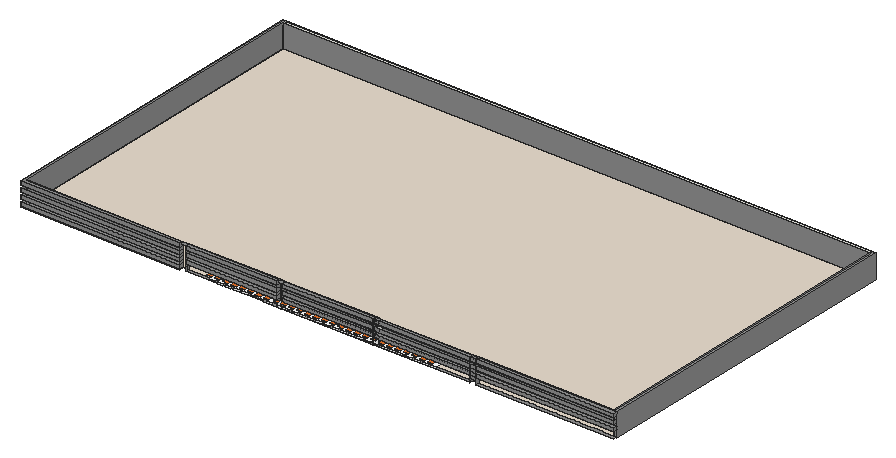
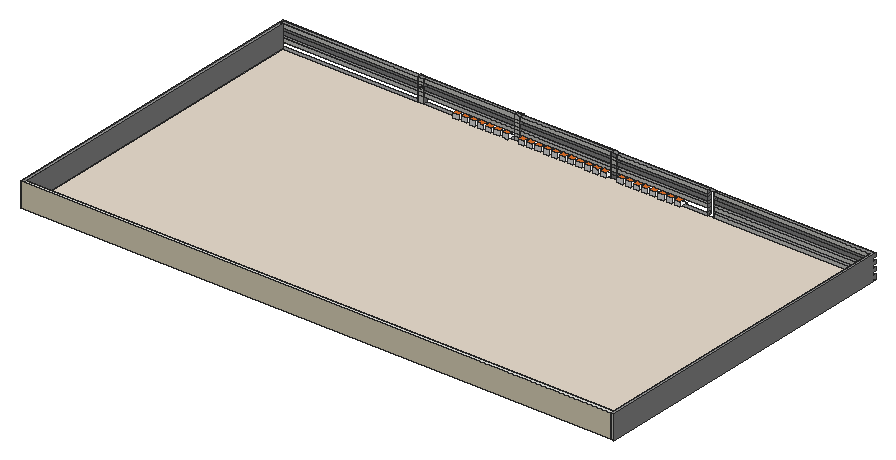
# SketchUp Ruby script. Lengths in inches.
U = 1.inch
M = Sketchup.active_model
def pt(a) = Geom::Point3d.new(a.map { |v| v * U })
def face(e, loops, mat)
  f = e.add_face(loops[0].map { |a| pt(a) })
  loops[1..].each { |l| e.add_face(l.map { |a| pt(a) }).erase! }
  f.material = f.back_material = mat if mat
  f
end
# faces: each face lists its corners as indices into pts; further lists are holes
def faces(e, pts, list, mat = nil) = list.each { |f| face(e, (f[0].is_a?(Array) ? f : [f]).map { |l| l.map { |i| pts[i] } }, mat) }
# xy, xz, yz: faces in a plane at the given z, y or x. An outline is a flat list of corners, or four numbers for a rectangle; further outlines are holes
def ring(l) = l.size == 4 ? [[l[0], l[1]], [l[2], l[1]], [l[2], l[3]], [l[0], l[3]]] : l.each_slice(2).to_a
def flat(e, list, mat, &to3) = list.each { |f| face(e, (f[0].is_a?(Array) ? f : [f]).map { |l| ring(l).map { |u, v| to3.(u, v) } }, mat) }
def xy(e, z, list, mat = nil) = flat(e, list, mat) { |x, y| [x, y, z] }
def xz(e, y, list, mat = nil) = flat(e, list, mat) { |x, z| [x, y, z] }
def yz(e, x, list, mat = nil) = flat(e, list, mat) { |y, z| [x, y, z] }
def lines(e, pts, list) = list.each { |a, b| e.add_line(pt(pts[a]), pt(pts[b])) }
# prism: a flat outline (further loops are holes) pulled along v
def prism(e, loops, v, mat = nil)
  f = face(e, loops, mat); d = Geom::Vector3d.new(v.map { |x| x * U })
  f.pushpull(f.normal.samedirection?(d) ? d.length : -d.length)
end
def box(e, o, s, mat = nil) = prism(e, [[o, [o[0] + s[0], o[1], o[2]], [o[0] + s[0], o[1] + s[1], o[2]], [o[0], o[1] + s[1], o[2]]]], [0, 0, s[2]], mat)
def at(x, y, z, deg = 0) = Geom::Transformation.translation(pt([x, y, z])) * Geom::Transformation.rotation(ORIGIN, Z_AXIS, deg.degrees)
def axes(o, x, y, z) = Geom::Transformation.new([*x, 0, *y, 0, *z, 0, *pt(o).to_a, 1])
def part(name) = M.definitions.add(name)
# library, detail: a bought-in or finely detailed component or shape, given as its bounding box
def library(name, o, s) = part(name).tap { |d| box(d.entities, o, s) }
def detail(e, o, s) = box(e.add_group.entities, o, s)
def put(e, d, t, mat = nil) = e.add_instance(d, t).tap { |i| i.material = mat if mat }
def group(e, t, mat = nil) = e.add_group.tap { |g| g.transformation = t; g.material = mat if mat }.entities
root = M.entities
M.materials.add("Generic").color = [146, 146, 146]
M.materials.add("Generic\#3").color = [226, 112, 41]
M.materials.add("Generic\#5").color = [249, 239, 211]
M.materials.add("Generic\#7").color = [232, 220, 205]
M.materials.add("[Color M00]").color = [255, 255, 255]
xy(root,1896.75,[[1505.875,322,1513,1033.625],[217.0625,1025.625,1505.875,1033.625]])
xy(root,1896.75,[[209.5,313.625,560.3,322],[209.5,322,217.0625,1033.625]],"Generic")
xy(root,1898.5625,[[773.9375,313.625,780.55,322]],"Generic")
xy(root,1899.375,[[572.47,313.625,737.9375,313.625,737.9375,314.3125,744.55,314.3125,744.55,313.625,772.57,313.625,772.57,322,572.47,322],[784.74,313.625,984.84,322],[997.01,313.625,1197.11,322],[1209.29,313.625,1513,322]],"Generic")
xy(root,1899.375,[[217.0625,322,1505.875,1025.625]],"Generic\#7")
xy(root,1902.875,[[624.9375,313.625,636.55,333.5625],[642.9375,313.625,654.55,333.5625],[660.9375,313.625,672.55,333.5625],[678.9375,313.625,690.55,333.5625],[696.9375,313.625,708.55,333.5625],
  [714.9375,313.625,726.55,333.5625],[732.9375,313.625,744.55,333.5625],[750.9375,313.625,762.55,333.5625],[786.9375,313.625,798.55,333.5625],[804.9375,313.625,816.55,333.5625],
  [822.9375,313.625,834.55,333.5625],[840.9375,313.625,852.55,333.5625],[858.9375,313.625,870.55,333.5625],[876.9375,313.625,888.55,333.5625],[894.9375,313.625,906.55,333.5625],
  [912.9375,313.625,924.55,333.5625],[930.9375,313.625,942.55,333.5625],[948.9375,313.625,960.55,333.5625],[966.9375,313.625,978.55,333.5625],[1002.9375,313.625,1014.55,333.5625],
  [1020.9375,313.625,1032.55,333.5625],[1038.9375,313.625,1050.55,333.5625],[1056.9375,313.625,1068.55,333.5625],[1074.9375,313.625,1086.55,333.5625],[1092.9375,313.625,1104.55,333.5625],
  [1110.9375,313.625,1122.55,333.5625]],"[Color M00]")
xy(root,1907.375,[[209.5,313.625,560.3,322]],"Generic")
xy(root,1913.3125,[[209.5,313.625,560.3,322],[572.47,313.625,624.9375,322],[624.9375,313.625,636.55,322],[636.55,313.625,642.9375,322],[642.9375,313.625,654.55,322],
  [654.55,313.625,660.9375,322],[660.9375,313.625,672.55,322],[672.55,313.625,678.9375,322],[678.9375,313.625,690.55,322],[690.55,313.625,696.9375,322],
  [696.9375,313.625,708.55,322],[708.55,313.625,714.9375,322],[714.9375,313.625,726.55,322],[726.55,313.625,732.9375,322],[732.9375,313.625,744.55,322],
  [744.55,313.625,750.9375,322],[750.9375,313.625,762.55,322],[762.55,313.625,772.57,322],[784.74,313.625,786.9375,322],[786.9375,313.625,798.55,322],
  [798.55,313.625,804.9375,322],[804.9375,313.625,816.55,322],[816.55,313.625,822.9375,322],[822.9375,313.625,834.55,322],[834.55,313.625,840.9375,322],
  [840.9375,313.625,852.55,322],[852.55,313.625,858.9375,322],[858.9375,313.625,870.55,322],[870.55,313.625,876.9375,322],[876.9375,313.625,888.55,322],
  [888.55,313.625,894.9375,322],[894.9375,313.625,906.55,322],[906.55,313.625,912.9375,322],[912.9375,313.625,924.55,322],[924.55,313.625,930.9375,322],
  [930.9375,313.625,942.55,322],[942.55,313.625,948.9375,322],[948.9375,313.625,960.55,322],[960.55,313.625,966.9375,322],[966.9375,313.625,978.55,322],
  [978.55,313.625,1002.9375,322],[1002.9375,313.625,1014.55,322],[1014.55,313.625,1020.9375,322],[1020.9375,313.625,1032.55,322],[1032.55,313.625,1038.9375,322],
  [1038.9375,313.625,1050.55,322],[1050.55,313.625,1056.9375,322],[1056.9375,313.625,1068.55,322],[1068.55,313.625,1074.9375,322],[1074.9375,313.625,1086.55,322],
  [1086.55,313.625,1092.9375,322],[1092.9375,313.625,1104.55,322],[1104.55,313.625,1110.9375,322],[1110.9375,313.625,1122.55,322],[1122.55,313.625,1513,322]],"Generic")
xy(root,1913.3125,[[732.9375,303.9375,744.55,313.625],[624.9375,305.625,636.55,313.625],[642.9375,305.625,654.55,313.625],[660.9375,305.625,672.55,313.625],[678.9375,305.625,690.55,313.625],
  [696.9375,305.625,708.55,313.625],[714.9375,305.625,726.55,313.625],[750.9375,305.625,762.55,313.625],[772.57,305.625,780.55,313.625],[786.9375,305.625,798.55,313.625],
  [804.9375,305.625,816.55,313.625],[822.9375,305.625,834.55,313.625],[840.9375,305.625,852.55,313.625],[858.9375,305.625,870.55,313.625],[876.9375,305.625,888.55,313.625],
  [894.9375,305.625,906.55,313.625],[912.9375,305.625,924.55,313.625],[930.9375,305.625,942.55,313.625],[948.9375,305.625,960.55,313.625],[966.9375,305.625,978.55,313.625],
  [984.9375,305.625,996.55,312.1875],[1002.9375,305.625,1014.55,313.625],[1020.9375,305.625,1032.55,313.625],[1038.9375,305.625,1050.55,313.625],[1056.9375,305.625,1068.55,313.625],
  [1074.9375,305.625,1086.55,313.625],[1092.9375,305.625,1104.55,313.625],[1110.9375,305.625,1122.55,313.625],[624.9375,322,636.55,333.5625],[642.9375,322,654.55,333.5625],
  [660.9375,322,672.55,333.5625],[678.9375,322,690.55,333.5625],[696.9375,322,708.55,333.5625],[714.9375,322,726.55,333.5625],[732.9375,322,744.55,333.5625],
  [750.9375,322,762.55,333.5625],[786.9375,322,798.55,333.5625],[804.9375,322,816.55,333.5625],[822.9375,322,834.55,333.5625],[840.9375,322,852.55,333.5625],
  [858.9375,322,870.55,333.5625],[876.9375,322,888.55,333.5625],[894.9375,322,906.55,333.5625],[912.9375,322,924.55,333.5625],[930.9375,322,942.55,333.5625],
  [948.9375,322,960.55,333.5625],[966.9375,322,978.55,333.5625],[1002.9375,322,1014.55,333.5625],[1020.9375,322,1032.55,333.5625],[1038.9375,322,1050.55,333.5625],
  [1056.9375,322,1068.55,333.5625],[1074.9375,322,1086.55,333.5625],[1092.9375,322,1104.55,333.5625],[1110.9375,322,1122.55,333.5625]],"Generic\#3")
xy(root,1921.3125,[[209.5,313.625,560.3,322],[572.47,313.625,772.57,322],[784.74,313.625,1513,322]],"Generic")
xy(root,1927.25,[[209.5,313.625,560.3,322],[572.47,313.625,772.57,322],[784.74,313.625,1513,322]],"Generic")
xy(root,1941.1875,[[209.5,313.625,560.3,322],[572.47,313.625,772.57,322],[784.74,313.625,1513,322]],"Generic")
xy(root,1949.1875,[[217.0625,1025.625,1505.875,1033.625]])
xy(root,1949.1875,[[984.84,312.1875,997.01,313.625],[1197.11,312.6875,1209.29,313.625],[209.5,313.625,560.3,313.625,560.3,322,217.0625,322,217.0625,1033.625,209.5,1033.625],[560.3,313.625,572.47,322],[572.47,313.625,772.57,322],
  [772.57,313.625,784.74,322],[784.74,313.625,984.84,322],[984.84,313.625,997.01,322],[997.01,313.625,1197.11,322],[1197.11,313.625,1209.29,322],
  [1209.29,313.625,1513,322],[1505.875,322,1513,1033.625]],"Generic")
xz(root,312.1875,[[984.9375,1902.875,996.55,1913.3125]],"[Color M00]")
xz(root,313.625,[[209.5,1899.375,560.3,1907.375],[984.84,1899.375,997.01,1907.375],[984.84,1907.375,997.01,1913.3125],[1197.11,1907.375,1209.29,1913.3125],[209.5,1913.3125,560.3,1921.3125],
  [572.47,1913.3125,772.57,1921.3125],[784.74,1913.3125,984.84,1921.3125],[984.84,1913.3125,997.01,1921.3125],[997.01,1913.3125,1197.11,1921.3125],[1197.11,1913.3125,1209.29,1921.3125],
  [1209.29,1913.3125,1513,1921.3125],[1197.11,1921.3125,1209.29,1927.25],[209.5,1927.25,560.3,1935.25],[572.47,1927.25,772.57,1935.25],[784.74,1927.25,984.84,1935.25],
  [984.84,1927.25,997.01,1935.25],[997.01,1927.25,1197.11,1935.25],[1197.11,1927.25,1209.29,1935.25],[1209.29,1927.25,1513,1935.25],[209.5,1941.1875,560.3,1949.1875],
  [572.47,1941.1875,772.57,1949.1875],[784.74,1941.1875,984.84,1949.1875],[984.84,1941.1875,997.01,1949.1875],[997.01,1941.1875,1197.11,1949.1875],[1197.11,1941.1875,1209.29,1949.1875],
  [1209.29,1941.1875,1513,1949.1875]],"Generic")
xz(root,313.625,[[772.57,1898.5625,780.55,1902.875],[624.9375,1899.375,636.55,1902.875],[642.9375,1899.375,654.55,1902.875],[660.9375,1899.375,672.55,1902.875],[678.9375,1899.375,690.55,1902.875],
  [696.9375,1899.375,708.55,1902.875],[714.9375,1899.375,726.55,1902.875],[750.9375,1899.375,762.55,1902.875],[786.9375,1899.375,798.55,1902.875],[804.9375,1899.375,816.55,1902.875],
  [822.9375,1899.375,834.55,1902.875],[840.9375,1899.375,852.55,1902.875],[858.9375,1899.375,870.55,1902.875],[876.9375,1899.375,888.55,1902.875],[894.9375,1899.375,906.55,1902.875],
  [912.9375,1899.375,924.55,1902.875],[930.9375,1899.375,942.55,1902.875],[948.9375,1899.375,960.55,1902.875],[966.9375,1899.375,978.55,1902.875],[1002.9375,1899.375,1014.55,1902.875],
  [1020.9375,1899.375,1032.55,1902.875],[1038.9375,1899.375,1050.55,1902.875],[1056.9375,1899.375,1068.55,1902.875],[1074.9375,1899.375,1086.55,1902.875],[1092.9375,1899.375,1104.55,1902.875],
  [1110.9375,1899.375,1122.55,1902.875],[772.57,1902.875,780.55,1913.3125]],"[Color M00]")
xz(root,322,[[217.0625,1899.375,560.3,1907.375],[984.84,1899.375,997.01,1907.375],[1197.11,1899.375,1209.29,1913.3125],[984.84,1907.375,997.01,1913.3125],[217.0625,1913.3125,560.3,1921.3125],
  [572.47,1913.3125,772.57,1921.3125],[772.57,1913.3125,784.74,1921.3125],[784.74,1913.3125,984.84,1921.3125],[984.84,1913.3125,997.01,1921.3125],[997.01,1913.3125,1197.11,1921.3125],
  [1197.11,1913.3125,1209.29,1921.3125],[1197.11,1913.3125,1209.29,1935.25],[1209.29,1913.3125,1505.875,1921.3125],[1505.875,1913.3125,1513,1921.3125],[984.84,1921.3125,997.01,1927.25],
  [984.84,1921.3125,997.01,1935.25],[1197.11,1921.3125,1209.29,1927.25],[772.57,1927.25,784.74,1935.25],[984.84,1927.25,997.01,1935.25],[1197.11,1927.25,1209.29,1935.25],
  [772.57,1935.25,784.74,1941.1875],[984.84,1935.25,997.01,1941.1875],[1197.11,1935.25,1209.29,1941.1875],[217.0625,1941.1875,560.3,1949.1875],[572.47,1941.1875,772.57,1949.1875],
  [784.74,1941.1875,984.84,1949.1875],[984.84,1941.1875,997.01,1949.1875],[997.01,1941.1875,1197.11,1949.1875],[1197.11,1941.1875,1209.29,1949.1875],[1209.29,1941.1875,1505.875,1949.1875],
  [1505.875,1941.1875,1513,1949.1875]])
xz(root,322,[[209.5,1896.75,217.0625,1899.375],[1505.875,1896.75,1513,1899.375],[772.57,1899.375,784.74,1907.375],[1505.875,1899.375,1513,1913.3125],[209.5,1907.375,217.0625,1913.3125],
  [772.57,1907.375,784.74,1913.3125],[209.5,1921.3125,217.0625,1927.25],[772.57,1921.3125,784.74,1927.25],[1505.875,1921.3125,1513,1927.25],[217.0625,1927.25,560.3,1935.25],
  [572.47,1927.25,772.57,1935.25],[784.74,1927.25,984.84,1935.25],[997.01,1927.25,1197.11,1935.25],[1209.29,1927.25,1505.875,1935.25],[1505.875,1927.25,1513,1941.1875],
  [209.5,1935.25,217.0625,1941.1875],[772.57,1941.1875,784.74,1949.1875]],"Generic")
xz(root,333.5625,[[624.9375,1902.875,636.55,1913.3125],[642.9375,1902.875,654.55,1913.3125],[660.9375,1902.875,672.55,1913.3125],[678.9375,1902.875,690.55,1913.3125],[696.9375,1902.875,708.55,1913.3125],
  [714.9375,1902.875,726.55,1913.3125],[732.9375,1902.875,744.55,1913.3125],[750.9375,1902.875,762.55,1913.3125],[786.9375,1902.875,798.55,1913.3125],[804.9375,1902.875,816.55,1913.3125],
  [822.9375,1902.875,834.55,1913.3125],[840.9375,1902.875,852.55,1913.3125],[858.9375,1902.875,870.55,1913.3125],[876.9375,1902.875,888.55,1913.3125],[894.9375,1902.875,906.55,1913.3125],
  [912.9375,1902.875,924.55,1913.3125],[930.9375,1902.875,942.55,1913.3125],[948.9375,1902.875,960.55,1913.3125],[966.9375,1902.875,978.55,1913.3125],[1002.9375,1902.875,1014.55,1913.3125],
  [1020.9375,1902.875,1032.55,1913.3125],[1038.9375,1902.875,1050.55,1913.3125],[1056.9375,1902.875,1068.55,1913.3125],[1074.9375,1902.875,1086.55,1913.3125],[1092.9375,1902.875,1104.55,1913.3125],
  [1110.9375,1902.875,1122.55,1913.3125]],"[Color M00]")
xz(root,1025.625,[[217.0625,1896.75,1505.875,1899.375]])
xz(root,1025.625,[[217.0625,1899.375,1505.875,1949.1875]],"Generic")
xz(root,1033.625,[[209.5,1896.75,217.0625,1949.1875]])
xz(root,1033.625,[[217.0625,1896.75,1513,1949.1875]],"Generic\#5")
yz(root,209.5,[[322,1896.75,322,1899.375,313.625,1899.375,313.625,1907.375,322,1907.375,322,1913.3125,313.625,1913.3125,313.625,1921.3125,322,1921.3125,322,1927.25,313.625,1927.25,313.625,1935.25,322,1935.25,322,1941.1875,313.625,1941.1875,313.625,1949.1875,1033.625,1949.1875,1033.625,1896.75]],"Generic")
yz(root,217.0625,[[1025.625,1896.75,1033.625,1949.1875]])
yz(root,217.0625,[[322,1896.75,1025.625,1899.375],[322,1899.375,1025.625,1949.1875]],"Generic")
yz(root,560.3,[[313.625,1896.75,322,1899.375],[313.625,1899.375,322,1907.375],[313.625,1907.375,322,1913.3125],[313.625,1913.3125,322,1921.3125],[313.625,1921.3125,322,1927.25],
  [313.625,1927.25,322,1935.25],[313.625,1935.25,322,1941.1875],[313.625,1941.1875,322,1949.1875]],"Generic")
yz(root,572.47,[[313.625,1899.375,315.625,1907.375],[315.625,1899.375,322,1907.375],[313.625,1907.375,322,1913.3125],[313.625,1913.3125,322,1921.3125],[313.625,1921.3125,322,1927.25],
  [313.625,1927.25,322,1935.25],[313.625,1935.25,322,1941.1875],[313.625,1941.1875,322,1949.1875]],"Generic")
yz(root,772.57,[[313.625,1899.375,315.625,1907.375],[315.625,1899.375,322,1907.375],[313.625,1907.375,322,1913.3125],[313.625,1913.3125,322,1921.3125],[313.625,1921.3125,322,1927.25],
  [313.625,1927.25,322,1935.25],[313.625,1935.25,322,1941.1875],[313.625,1941.1875,322,1949.1875]],"Generic")
yz(root,784.74,[[313.625,1899.375,322,1907.375],[313.625,1907.375,322,1913.3125],[313.625,1913.3125,322,1921.3125],[313.625,1921.3125,322,1927.25],[313.625,1927.25,322,1935.25],
  [313.625,1935.25,322,1941.1875],[313.625,1941.1875,322,1949.1875]],"Generic")
yz(root,984.84,[[312.1875,1899.375,313.625,1907.375],[313.625,1899.375,322,1949.1875],[312.1875,1907.375,313.625,1913.3125],[312.1875,1913.3125,313.625,1921.3125],[312.1875,1921.3125,313.625,1927.25],
  [312.1875,1927.25,313.625,1935.25],[312.1875,1935.25,313.625,1941.1875],[312.1875,1941.1875,313.625,1949.1875]],"Generic")
yz(root,1197.11,[[312.6875,1899.375,313.625,1907.375],[313.625,1899.375,313.625,1935.25,312.6875,1935.25,312.6875,1941.1875,313.625,1941.1875,313.625,1949.1875,322,1949.1875,322,1899.375],[312.6875,1907.375,313.625,1913.3125],[312.6875,1913.3125,313.625,1921.3125],[312.6875,1921.3125,313.625,1927.25],
  [312.6875,1927.25,313.625,1935.25],[312.6875,1941.1875,313.625,1949.1875]],"Generic")
yz(root,1209.29,[[312.6875,1899.375,322,1949.1875]],"Generic")
yz(root,1505.875,[[322,1896.75,1025.625,1899.375]])
yz(root,1505.875,[[322,1899.375,1025.625,1949.1875]],"Generic")
yz(root,1513,[[322,1896.75,1033.625,1949.1875],[313.625,1913.3125,322,1921.3125],[313.625,1927.25,322,1935.25],[313.625,1941.1875,322,1949.1875]],"Generic")
p = [[560.3,322,1941.1875],[572.47,322,1941.1875],[560.3,322,1935.25],[572.47,322,1935.25],[560.3,322,1927.25],[572.47,322,1927.25],
  [560.3,322,1921.3125],[572.47,322,1921.3125],[560.3,322,1913.3125],[572.47,322,1913.3125],[560.3,322,1907.375],[572.47,322,1907.375]]
lines(root,p,[[0,1],[2,3],[4,5],[6,7],[8,9],[10,11]])
